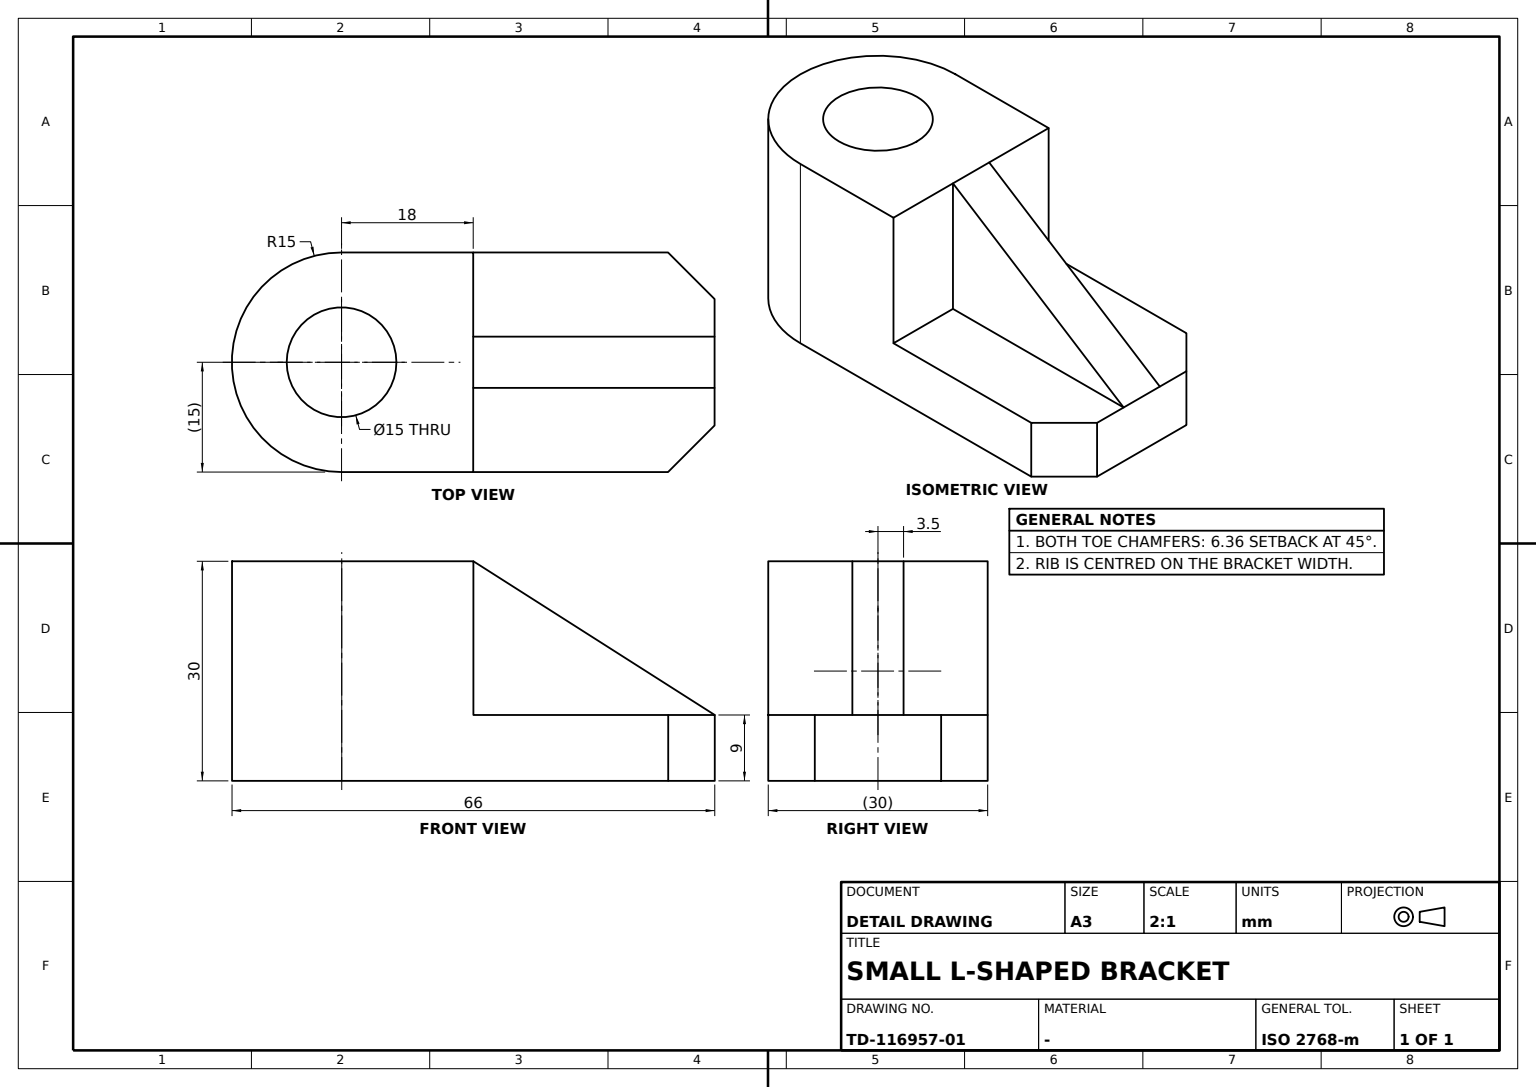
ISO-10303-21;
HEADER;
FILE_DESCRIPTION((''),'2;1');
FILE_NAME('','',(''),(''),'','','');
FILE_SCHEMA(('AUTOMOTIVE_DESIGN'));
ENDSEC;
DATA;
#1=APPLICATION_CONTEXT('');
#2=PRODUCT_CONTEXT('',#1,'mechanical');
#3=PRODUCT('','','',(#2));
#4=PRODUCT_DEFINITION_FORMATION('','',#3);
#5=PRODUCT_DEFINITION_CONTEXT('',#1,'design');
#6=PRODUCT_DEFINITION('','',#4,#5);
#7=PRODUCT_DEFINITION_SHAPE('','',#6);
#8=(LENGTH_UNIT()NAMED_UNIT(*)SI_UNIT(.MILLI.,.METRE.));
#9=(NAMED_UNIT(*)PLANE_ANGLE_UNIT()SI_UNIT($,.RADIAN.));
#10=(NAMED_UNIT(*)SI_UNIT($,.STERADIAN.)SOLID_ANGLE_UNIT());
#11=UNCERTAINTY_MEASURE_WITH_UNIT(LENGTH_MEASURE(0.005),#8,'distance_accuracy_value','');
#12=(GEOMETRIC_REPRESENTATION_CONTEXT(3)GLOBAL_UNCERTAINTY_ASSIGNED_CONTEXT((#11))GLOBAL_UNIT_ASSIGNED_CONTEXT((#8,#9,#10))REPRESENTATION_CONTEXT('',''));
#13=CARTESIAN_POINT('',(33.,-3.5,9.));
#14=VERTEX_POINT('',#13);
#15=CARTESIAN_POINT('',(33.,3.5,9.));
#16=VERTEX_POINT('',#15);
#17=CARTESIAN_POINT('',(33.,-8.636039,9.));
#18=DIRECTION('',(0.,1.,0.));
#19=VECTOR('',#18,1000.);
#20=LINE('',#17,#19);
#21=EDGE_CURVE('',#14,#16,#20,.T.);
#22=ORIENTED_EDGE('',*,*,#21,.T.);
#23=CARTESIAN_POINT('',(0.,3.5,30.));
#24=VERTEX_POINT('',#23);
#25=CARTESIAN_POINT('',(13.588235,3.5,21.352941));
#26=DIRECTION('',(-0.843661488,0.,0.536875492));
#27=VECTOR('',#26,1000.);
#28=LINE('',#25,#27);
#29=EDGE_CURVE('',#16,#24,#28,.T.);
#30=ORIENTED_EDGE('',*,*,#29,.T.);
#31=CARTESIAN_POINT('',(0.,-3.5,30.));
#32=VERTEX_POINT('',#31);
#33=CARTESIAN_POINT('',(0.,0.,30.));
#34=LINE('',#33,#19);
#35=EDGE_CURVE('',#32,#24,#34,.T.);
#36=ORIENTED_EDGE('',*,*,#35,.F.);
#37=CARTESIAN_POINT('',(13.588235,-3.5,21.352941));
#38=LINE('',#37,#27);
#39=EDGE_CURVE('',#14,#32,#38,.T.);
#40=ORIENTED_EDGE('',*,*,#39,.F.);
#41=EDGE_LOOP('',(#22,#30,#36,#40));
#42=FACE_BOUND('',#41,.T.);
#43=CARTESIAN_POINT('',(33.,0.,9.));
#44=DIRECTION('',(-0.536875492,0.,-0.843661488));
#45=AXIS2_PLACEMENT_3D('',#43,#44,#26);
#46=PLANE('',#45);
#47=ADVANCED_FACE('',(#42),#46,.F.);
#48=CARTESIAN_POINT('',(33.,-8.636039,0.));
#49=VERTEX_POINT('',#48);
#50=CARTESIAN_POINT('',(33.,8.636039,0.));
#51=VERTEX_POINT('',#50);
#52=CARTESIAN_POINT('',(33.,0.,0.));
#53=LINE('',#52,#19);
#54=EDGE_CURVE('',#49,#51,#53,.T.);
#55=ORIENTED_EDGE('',*,*,#54,.T.);
#56=CARTESIAN_POINT('',(33.,8.636039,9.));
#57=VERTEX_POINT('',#56);
#58=DIRECTION('',(0.,0.,1.));
#59=VECTOR('',#58,1000.);
#60=LINE('',#50,#59);
#61=EDGE_CURVE('',#51,#57,#60,.T.);
#62=ORIENTED_EDGE('',*,*,#61,.T.);
#63=LINE('',#43,#19);
#64=EDGE_CURVE('',#16,#57,#63,.T.);
#65=ORIENTED_EDGE('',*,*,#64,.F.);
#66=ORIENTED_EDGE('',*,*,#21,.F.);
#67=VERTEX_POINT('',#17);
#68=EDGE_CURVE('',#67,#14,#63,.T.);
#69=ORIENTED_EDGE('',*,*,#68,.F.);
#70=LINE('',#48,#59);
#71=EDGE_CURVE('',#49,#67,#70,.T.);
#72=ORIENTED_EDGE('',*,*,#71,.F.);
#73=EDGE_LOOP('',(#55,#62,#65,#66,#69,#72));
#74=FACE_BOUND('',#73,.T.);
#75=DIRECTION('',(1.,0.,0.));
#76=AXIS2_PLACEMENT_3D('',#48,#75,#18);
#77=PLANE('',#76);
#78=ADVANCED_FACE('',(#74),#77,.T.);
#79=CARTESIAN_POINT('',(0.,3.5,9.));
#80=VERTEX_POINT('',#79);
#81=CARTESIAN_POINT('',(0.,3.5,0.));
#82=DIRECTION('',(0.,0.,-1.));
#83=VECTOR('',#82,1000.);
#84=LINE('',#81,#83);
#85=EDGE_CURVE('',#24,#80,#84,.T.);
#86=ORIENTED_EDGE('',*,*,#85,.F.);
#87=ORIENTED_EDGE('',*,*,#29,.F.);
#88=VECTOR('',#75,1000.);
#89=LINE('',#79,#88);
#90=EDGE_CURVE('',#80,#16,#89,.T.);
#91=ORIENTED_EDGE('',*,*,#90,.F.);
#92=EDGE_LOOP('',(#86,#87,#91));
#93=FACE_BOUND('',#92,.T.);
#94=DIRECTION('',(-1.,0.,0.));
#95=AXIS2_PLACEMENT_3D('',#81,#18,#94);
#96=PLANE('',#95);
#97=ADVANCED_FACE('',(#93),#96,.T.);
#98=CARTESIAN_POINT('',(0.,-3.5,9.));
#99=VERTEX_POINT('',#98);
#100=CARTESIAN_POINT('',(0.,-15.,9.));
#101=VERTEX_POINT('',#100);
#102=CARTESIAN_POINT('',(0.,0.,9.));
#103=DIRECTION('',(0.,-1.,0.));
#104=VECTOR('',#103,1000.);
#105=LINE('',#102,#104);
#106=EDGE_CURVE('',#99,#101,#105,.T.);
#107=ORIENTED_EDGE('',*,*,#106,.T.);
#108=CARTESIAN_POINT('',(26.636039,-15.,9.));
#109=VERTEX_POINT('',#108);
#110=VECTOR('',#94,1000.);
#111=LINE('',#100,#110);
#112=EDGE_CURVE('',#109,#101,#111,.T.);
#113=ORIENTED_EDGE('',*,*,#112,.F.);
#114=CARTESIAN_POINT('',(20.818019,-20.818019,9.));
#115=DIRECTION('',(-0.707106781,-0.707106781,0.));
#116=VECTOR('',#115,1000.);
#117=LINE('',#114,#116);
#118=EDGE_CURVE('',#67,#109,#117,.T.);
#119=ORIENTED_EDGE('',*,*,#118,.F.);
#120=ORIENTED_EDGE('',*,*,#68,.T.);
#121=LINE('',#98,#88);
#122=EDGE_CURVE('',#99,#14,#121,.T.);
#123=ORIENTED_EDGE('',*,*,#122,.F.);
#124=EDGE_LOOP('',(#107,#113,#119,#120,#123));
#125=FACE_BOUND('',#124,.T.);
#126=AXIS2_PLACEMENT_3D('',#102,#58,#75);
#127=PLANE('',#126);
#128=ADVANCED_FACE('',(#125),#127,.T.);
#129=CARTESIAN_POINT('',(-18.,-15.,0.));
#130=VERTEX_POINT('',#129);
#131=CARTESIAN_POINT('',(-18.,-15.,30.));
#132=VERTEX_POINT('',#131);
#133=CARTESIAN_POINT('',(-18.,-15.,15.));
#134=LINE('',#133,#59);
#135=EDGE_CURVE('',#130,#132,#134,.T.);
#136=ORIENTED_EDGE('',*,*,#135,.F.);
#137=CARTESIAN_POINT('',(26.636039,-15.,0.));
#138=VERTEX_POINT('',#137);
#139=CARTESIAN_POINT('',(0.,-15.,0.));
#140=LINE('',#139,#110);
#141=EDGE_CURVE('',#138,#130,#140,.T.);
#142=ORIENTED_EDGE('',*,*,#141,.F.);
#143=LINE('',#137,#59);
#144=EDGE_CURVE('',#138,#109,#143,.T.);
#145=ORIENTED_EDGE('',*,*,#144,.T.);
#146=ORIENTED_EDGE('',*,*,#112,.T.);
#147=CARTESIAN_POINT('',(0.,-15.,30.));
#148=VERTEX_POINT('',#147);
#149=LINE('',#139,#59);
#150=EDGE_CURVE('',#101,#148,#149,.T.);
#151=ORIENTED_EDGE('',*,*,#150,.T.);
#152=LINE('',#147,#110);
#153=EDGE_CURVE('',#148,#132,#152,.T.);
#154=ORIENTED_EDGE('',*,*,#153,.T.);
#155=EDGE_LOOP('',(#136,#142,#145,#146,#151,#154));
#156=FACE_BOUND('',#155,.T.);
#157=AXIS2_PLACEMENT_3D('',#139,#18,#94);
#158=PLANE('',#157);
#159=ADVANCED_FACE('',(#156),#158,.F.);
#160=CARTESIAN_POINT('',(0.,15.,30.));
#161=VERTEX_POINT('',#160);
#162=LINE('',#33,#104);
#163=EDGE_CURVE('',#161,#24,#162,.T.);
#164=ORIENTED_EDGE('',*,*,#163,.F.);
#165=CARTESIAN_POINT('',(-18.,15.,30.));
#166=VERTEX_POINT('',#165);
#167=LINE('',#160,#88);
#168=EDGE_CURVE('',#166,#161,#167,.T.);
#169=ORIENTED_EDGE('',*,*,#168,.F.);
#170=CARTESIAN_POINT('',(-18.,0.,30.));
#171=AXIS2_PLACEMENT_3D('',#170,#58,#75);
#172=CIRCLE('',#171,15.);
#173=EDGE_CURVE('',#166,#132,#172,.T.);
#174=ORIENTED_EDGE('',*,*,#173,.T.);
#175=ORIENTED_EDGE('',*,*,#153,.F.);
#176=EDGE_CURVE('',#32,#148,#162,.T.);
#177=ORIENTED_EDGE('',*,*,#176,.F.);
#178=ORIENTED_EDGE('',*,*,#35,.T.);
#179=EDGE_LOOP('',(#164,#169,#174,#175,#177,#178));
#180=FACE_BOUND('',#179,.T.);
#181=CARTESIAN_POINT('',(-10.5,0.,30.));
#182=VERTEX_POINT('',#181);
#183=CIRCLE('',#171,7.5);
#184=EDGE_CURVE('',#182,#182,#183,.T.);
#185=ORIENTED_EDGE('',*,*,#184,.F.);
#186=EDGE_LOOP('',(#185));
#187=FACE_BOUND('',#186,.T.);
#188=AXIS2_PLACEMENT_3D('',#33,#58,#75);
#189=PLANE('',#188);
#190=ADVANCED_FACE('',(#180,#187),#189,.T.);
#191=CARTESIAN_POINT('',(0.,15.,9.));
#192=VERTEX_POINT('',#191);
#193=CARTESIAN_POINT('',(26.636039,15.,9.));
#194=VERTEX_POINT('',#193);
#195=LINE('',#191,#88);
#196=EDGE_CURVE('',#192,#194,#195,.T.);
#197=ORIENTED_EDGE('',*,*,#196,.T.);
#198=CARTESIAN_POINT('',(26.636039,15.,0.));
#199=VERTEX_POINT('',#198);
#200=LINE('',#198,#59);
#201=EDGE_CURVE('',#199,#194,#200,.T.);
#202=ORIENTED_EDGE('',*,*,#201,.F.);
#203=CARTESIAN_POINT('',(-18.,15.,0.));
#204=VERTEX_POINT('',#203);
#205=CARTESIAN_POINT('',(0.,15.,0.));
#206=LINE('',#205,#88);
#207=EDGE_CURVE('',#204,#199,#206,.T.);
#208=ORIENTED_EDGE('',*,*,#207,.F.);
#209=CARTESIAN_POINT('',(-18.,15.,15.));
#210=LINE('',#209,#59);
#211=EDGE_CURVE('',#204,#166,#210,.T.);
#212=ORIENTED_EDGE('',*,*,#211,.T.);
#213=ORIENTED_EDGE('',*,*,#168,.T.);
#214=LINE('',#205,#59);
#215=EDGE_CURVE('',#192,#161,#214,.T.);
#216=ORIENTED_EDGE('',*,*,#215,.F.);
#217=EDGE_LOOP('',(#197,#202,#208,#212,#213,#216));
#218=FACE_BOUND('',#217,.T.);
#219=AXIS2_PLACEMENT_3D('',#203,#103,#75);
#220=PLANE('',#219);
#221=ADVANCED_FACE('',(#218),#220,.F.);
#222=CARTESIAN_POINT('',(-18.,0.,0.));
#223=AXIS2_PLACEMENT_3D('',#222,#58,#75);
#224=CIRCLE('',#223,15.);
#225=EDGE_CURVE('',#204,#130,#224,.T.);
#226=ORIENTED_EDGE('',*,*,#225,.T.);
#227=ORIENTED_EDGE('',*,*,#135,.T.);
#228=ORIENTED_EDGE('',*,*,#173,.F.);
#229=ORIENTED_EDGE('',*,*,#211,.F.);
#230=EDGE_LOOP('',(#226,#227,#228,#229));
#231=FACE_BOUND('',#230,.T.);
#232=CARTESIAN_POINT('',(-18.,0.,15.));
#233=AXIS2_PLACEMENT_3D('',#232,#58,#75);
#234=CYLINDRICAL_SURFACE('',#233,15.);
#235=ADVANCED_FACE('',(#231),#234,.T.);
#236=CARTESIAN_POINT('',(20.818019,20.818019,0.));
#237=DIRECTION('',(0.707106781,-0.707106781,0.));
#238=VECTOR('',#237,1000.);
#239=LINE('',#236,#238);
#240=EDGE_CURVE('',#199,#51,#239,.T.);
#241=ORIENTED_EDGE('',*,*,#240,.F.);
#242=ORIENTED_EDGE('',*,*,#201,.T.);
#243=CARTESIAN_POINT('',(20.818019,20.818019,9.));
#244=LINE('',#243,#238);
#245=EDGE_CURVE('',#194,#57,#244,.T.);
#246=ORIENTED_EDGE('',*,*,#245,.T.);
#247=ORIENTED_EDGE('',*,*,#61,.F.);
#248=EDGE_LOOP('',(#241,#242,#246,#247));
#249=FACE_BOUND('',#248,.T.);
#250=AXIS2_PLACEMENT_3D('',#198,#115,#237);
#251=PLANE('',#250);
#252=ADVANCED_FACE('',(#249),#251,.F.);
#253=ORIENTED_EDGE('',*,*,#184,.T.);
#254=EDGE_LOOP('',(#253));
#255=FACE_BOUND('',#254,.T.);
#256=CARTESIAN_POINT('',(-10.5,0.,0.));
#257=VERTEX_POINT('',#256);
#258=CIRCLE('',#223,7.5);
#259=EDGE_CURVE('',#257,#257,#258,.T.);
#260=ORIENTED_EDGE('',*,*,#259,.F.);
#261=EDGE_LOOP('',(#260));
#262=FACE_BOUND('',#261,.T.);
#263=CYLINDRICAL_SURFACE('',#233,7.5);
#264=ADVANCED_FACE('',(#255,#262),#263,.F.);
#265=ORIENTED_EDGE('',*,*,#106,.F.);
#266=CARTESIAN_POINT('',(0.,-3.5,0.));
#267=LINE('',#266,#83);
#268=EDGE_CURVE('',#32,#99,#267,.T.);
#269=ORIENTED_EDGE('',*,*,#268,.F.);
#270=ORIENTED_EDGE('',*,*,#176,.T.);
#271=ORIENTED_EDGE('',*,*,#150,.F.);
#272=EDGE_LOOP('',(#265,#269,#270,#271));
#273=FACE_BOUND('',#272,.T.);
#274=AXIS2_PLACEMENT_3D('',#205,#94,#103);
#275=PLANE('',#274);
#276=ADVANCED_FACE('',(#273),#275,.F.);
#277=ORIENTED_EDGE('',*,*,#196,.F.);
#278=EDGE_CURVE('',#192,#80,#105,.T.);
#279=ORIENTED_EDGE('',*,*,#278,.T.);
#280=ORIENTED_EDGE('',*,*,#90,.T.);
#281=ORIENTED_EDGE('',*,*,#64,.T.);
#282=ORIENTED_EDGE('',*,*,#245,.F.);
#283=EDGE_LOOP('',(#277,#279,#280,#281,#282));
#284=FACE_BOUND('',#283,.T.);
#285=ADVANCED_FACE('',(#284),#127,.T.);
#286=ORIENTED_EDGE('',*,*,#144,.F.);
#287=CARTESIAN_POINT('',(20.818019,-20.818019,0.));
#288=LINE('',#287,#116);
#289=EDGE_CURVE('',#49,#138,#288,.T.);
#290=ORIENTED_EDGE('',*,*,#289,.F.);
#291=ORIENTED_EDGE('',*,*,#71,.T.);
#292=ORIENTED_EDGE('',*,*,#118,.T.);
#293=EDGE_LOOP('',(#286,#290,#291,#292));
#294=FACE_BOUND('',#293,.T.);
#295=DIRECTION('',(-0.707106781,0.707106781,0.));
#296=AXIS2_PLACEMENT_3D('',#48,#295,#115);
#297=PLANE('',#296);
#298=ADVANCED_FACE('',(#294),#297,.F.);
#299=ORIENTED_EDGE('',*,*,#141,.T.);
#300=ORIENTED_EDGE('',*,*,#225,.F.);
#301=ORIENTED_EDGE('',*,*,#207,.T.);
#302=ORIENTED_EDGE('',*,*,#240,.T.);
#303=ORIENTED_EDGE('',*,*,#54,.F.);
#304=ORIENTED_EDGE('',*,*,#289,.T.);
#305=EDGE_LOOP('',(#299,#300,#301,#302,#303,#304));
#306=FACE_BOUND('',#305,.T.);
#307=ORIENTED_EDGE('',*,*,#259,.T.);
#308=EDGE_LOOP('',(#307));
#309=FACE_BOUND('',#308,.T.);
#310=CARTESIAN_POINT('',(0.,0.,0.));
#311=AXIS2_PLACEMENT_3D('',#310,#58,#75);
#312=PLANE('',#311);
#313=ADVANCED_FACE('',(#306,#309),#312,.F.);
#314=ORIENTED_EDGE('',*,*,#39,.T.);
#315=ORIENTED_EDGE('',*,*,#268,.T.);
#316=ORIENTED_EDGE('',*,*,#122,.T.);
#317=EDGE_LOOP('',(#314,#315,#316));
#318=FACE_BOUND('',#317,.T.);
#319=AXIS2_PLACEMENT_3D('',#266,#18,#94);
#320=PLANE('',#319);
#321=ADVANCED_FACE('',(#318),#320,.F.);
#322=ORIENTED_EDGE('',*,*,#163,.T.);
#323=ORIENTED_EDGE('',*,*,#85,.T.);
#324=ORIENTED_EDGE('',*,*,#278,.F.);
#325=ORIENTED_EDGE('',*,*,#215,.T.);
#326=EDGE_LOOP('',(#322,#323,#324,#325));
#327=FACE_BOUND('',#326,.T.);
#328=ADVANCED_FACE('',(#327),#275,.F.);
#329=CLOSED_SHELL('',(#47,#78,#97,#128,#159,#190,#221,#235,#252,#264,#276,#285,#298,#313,#321,#328));
#330=MANIFOLD_SOLID_BREP('',#329);
#331=ADVANCED_BREP_SHAPE_REPRESENTATION('',(#330),#12);
#332=SHAPE_DEFINITION_REPRESENTATION(#7,#331);
ENDSEC;
END-ISO-10303-21;
